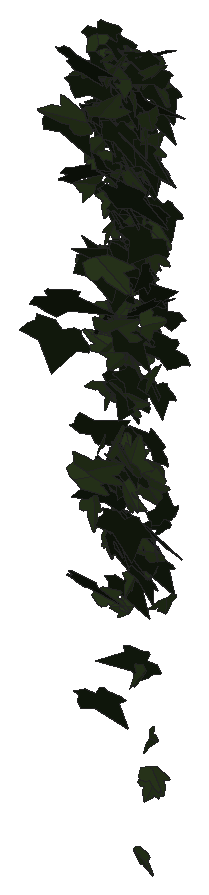
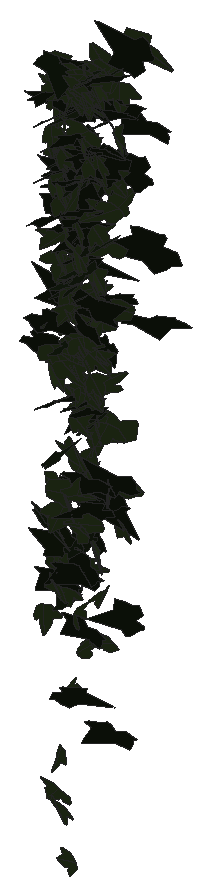
# SketchUp Ruby script. Lengths in millimetres.
U = 1.mm
M = Sketchup.active_model
def pt(a) = Geom::Point3d.new(a.map { |v| v * U })
def face(e, loops, mat)
  f = e.add_face(loops[0].map { |a| pt(a) })
  loops[1..].each { |l| e.add_face(l.map { |a| pt(a) }).erase! }
  f.material = f.back_material = mat if mat
  f
end
# faces: each face lists its corners as indices into pts; further lists are holes
def faces(e, pts, list, mat = nil) = list.each { |f| face(e, (f[0].is_a?(Array) ? f : [f]).map { |l| l.map { |i| pts[i] } }, mat) }
# xy, xz, yz: faces in a plane at the given z, y or x. An outline is a flat list of corners, or four numbers for a rectangle; further outlines are holes
def ring(l) = l.size == 4 ? [[l[0], l[1]], [l[2], l[1]], [l[2], l[3]], [l[0], l[3]]] : l.each_slice(2).to_a
def flat(e, list, mat, &to3) = list.each { |f| face(e, (f[0].is_a?(Array) ? f : [f]).map { |l| ring(l).map { |u, v| to3.(u, v) } }, mat) }
def xy(e, z, list, mat = nil) = flat(e, list, mat) { |x, y| [x, y, z] }
def xz(e, y, list, mat = nil) = flat(e, list, mat) { |x, z| [x, y, z] }
def yz(e, x, list, mat = nil) = flat(e, list, mat) { |y, z| [x, y, z] }
def lines(e, pts, list) = list.each { |a, b| e.add_line(pt(pts[a]), pt(pts[b])) }
# prism: a flat outline (further loops are holes) pulled along v
def prism(e, loops, v, mat = nil)
  f = face(e, loops, mat); d = Geom::Vector3d.new(v.map { |x| x * U })
  f.pushpull(f.normal.samedirection?(d) ? d.length : -d.length)
end
def box(e, o, s, mat = nil) = prism(e, [[o, [o[0] + s[0], o[1], o[2]], [o[0] + s[0], o[1] + s[1], o[2]], [o[0], o[1] + s[1], o[2]]]], [0, 0, s[2]], mat)
def at(x, y, z, deg = 0) = Geom::Transformation.translation(pt([x, y, z])) * Geom::Transformation.rotation(ORIGIN, Z_AXIS, deg.degrees)
def axes(o, x, y, z) = Geom::Transformation.new([*x, 0, *y, 0, *z, 0, *pt(o).to_a, 1])
def part(name) = M.definitions.add(name)
# library, detail: a bought-in or finely detailed component or shape, given as its bounding box
def library(name, o, s) = part(name).tap { |d| box(d.entities, o, s) }
def detail(e, o, s) = box(e.add_group.entities, o, s)
def put(e, d, t, mat = nil) = e.add_instance(d, t).tap { |i| i.material = mat if mat }
def group(e, t, mat = nil) = e.add_group.tap { |g| g.transformation = t; g.material = mat if mat }.entities
root = M.entities
M.materials.add("efeu1").color = [18, 25, 13]
M.materials.add("efeu2").color = [43, 57, 29]
c1 = part("ivyleaf_9")
p = [[39.1,54.8,31.7],[34.5,51.8,30.2],[-5.3,25.2,17.3],[-17.9,28.3,20.9],[-21.6,21.7,17],[-20.2,4.3,5.3],
  [-22.9,-0.3,2.5],[-17.1,-4,-0.6],[-2,-2.1,-1.2],[-0.7,-15.4,-10.1],[16.6,-22.3,-16.7],[21.1,-15.1,-12.5],
  [32.7,-10.7,-11],[46.1,-1.8,-6.6],[30.8,11.2,3.8]]
faces(c1.entities,p,[[0,1,2,3,4,5,6,7,8,9,10,11,12,13,14]],"efeu1")
c2 = part("ivyleaf_10")
p = [[0,12.8,-0.8],[-1.5,51.3,-10.9],[-4.9,51,-11.6],[-13.6,26.5,-7.3],[-13.2,15.9,-4.6],[-21.1,19.3,-7.2],
  [-29.5,16.3,-8.3],[-29.2,8.3,-6.2],[-19.7,-9.8,0.5],[-7.6,-13,4],[1,-12.2,5.8],[-0.4,51.1,-11.1],
  [-1.5,51.1,-10.9],[1,-12.4,5.9],[16.9,-12.4,3.5],[35.1,9.1,-5.1],[35,12.9,-6.1],[20.5,16.4,-4.9],
  [15.8,15,-3.8],[15.3,27.6,-7.1],[12.8,31.3,-7.8]]
faces(c2.entities,p,[[0,1,2,3,4,5,6,7,8,9,10],[11,12,0,13,14,15,16,17,18,19,20]],"efeu2")
put(root,c1,axes([1553.2,964.1,820.5],[-0.50844,0.05858,0.77802],[1.40559,-0.24621,0.27213],[0.47885,0.7849,0.02729]))
put(root,c2,axes([1579.3,950.2,1427.7],[-0.24843,-0.69259,0.43871],[-0.02175,-0.44266,-0.70222],[1.56018,-0.11645,0.06007]))
put(root,c2,axes([1577,960.7,824.2],[0.33546,-0.65964,-0.42013],[0.02498,0.43311,-0.6745],[1.48823,0.14142,0.10602]))
put(root,c1,axes([1546.8,926.5,544.2],[1.31033,-0.2504,0.31362],[0.56981,-0.09424,-0.7325],[0.50862,0.75066,0.01266]))
put(root,c2,axes([1580.3,922.5,1594.3],[-0.565,-0.7823,-0.20791],[0.09233,0.20386,-0.83633],[1.5378,-0.29967,-0.02617]))
put(root,c2,axes([1573.2,980.5,613.6],[0.08437,0.74047,-0.08975],[-0.02204,-0.08921,-0.74177],[-1.4194,0.0454,0.00618]))
put(root,c2,axes([1580,985.8,1246.2],[0.21882,-0.71346,0.22089],[0.15293,-0.21038,-0.72134],[1.4132,0.13324,0.04385]))
put(root,c1,axes([1569.5,984.6,1311.2],[-0.05011,-0.74368,0.2109],[-0.00636,-0.21091,-0.74413],[1.47117,-0.02624,0.00397]))
put(root,c2,axes([1587.5,986.1,1080.6],[-0.54365,-0.54241,0.47693],[-0.09608,-0.49662,-0.59505],[1.37126,-0.24984,0.14739]))
put(root,c2,axes([1576.9,950,1631.2],[0.52706,0.80701,-0.11706],[-0.07471,-0.11029,-0.8532],[-1.55018,0.2797,0.00132]))
put(root,c2,axes([1553.1,947.1,1170.7],[0.32062,-0.03138,-0.82619],[1.5099,0.24348,0.15252],[0.44293,-0.80727,0.07812]))
put(root,c2,axes([1578.4,932.1,1503.4],[0.49586,-0.68935,0.42023],[0.32415,-0.3847,-0.73667],[1.50195,0.31061,0.02025]))
put(root,c2,axes([1587.8,921.2,1357],[-0.25254,-0.35305,-0.84263],[-0.52564,-0.79613,0.37706],[-1.65742,0.30628,0.00881]))
put(root,c2,axes([1563,971.4,1378.3],[0.66493,0.37712,0.69187],[0.69454,0.59333,-0.50769],[-1.32915,0.4987,0.08083]))
put(root,c2,axes([1594.5,961.7,1014.7],[0.50491,0.5468,0.55529],[-0.49909,-0.48974,0.60754],[1.3967,-0.37267,0.01636]))
put(root,c1,axes([1607.6,969.1,1162.5],[0.25194,0.01031,0.85113],[-1.24923,0.54964,0.09543],[-1.03139,-0.6632,0.09232]))
put(root,c1,axes([1581.6,836.9,1095.2],[-1.20945,-0.79383,-0.19057],[0.21871,0.15212,-1.01684],[1.53827,-0.64577,-0.00526]))
put(root,c2,axes([1581.3,963.3,931],[-1.14052,-0.32781,-0.19698],[0.35024,0.07381,-0.68269],[0.63805,-0.62647,0.02264]))
put(root,c1,axes([1553.1,970.7,1466.3],[0.51611,-0.04869,0.76965],[1.46731,-0.00217,-0.27178],[0.0347,0.81602,0.0452]))
put(root,c1,axes([1565.5,966.3,1642.5],[0.4766,-0.57612,-0.54841],[0.17839,0.59232,-0.57945],[1.50328,0.11237,0.24263]))
put(root,c2,axes([1589.3,978.5,1474.5],[0.98995,-0.60809,-0.19504],[-0.1747,0.17774,-0.79897],[1.20277,0.52631,0.04448]))
put(root,c2,axes([1589.2,991.4,1471.5],[-0.44788,-0.6787,0.35841],[0.07888,-0.38557,-0.70291],[1.45861,-0.18755,0.14807]))
put(root,c2,axes([1590,984.7,1035],[-0.28456,-0.65758,0.24603],[0.0679,-0.25834,-0.6688],[1.33451,-0.12707,0.08649]))
put(root,c1,axes([1568.6,867.1,1511],[-0.737,-0.30191,-0.75298],[1.19702,0.41527,-0.48996],[0.97519,-0.7379,0.03234]))
put(root,c1,axes([1568.7,953.4,1464],[0.3838,-0.72001,0.34686],[0.20512,-0.32996,-0.7476],[1.50715,0.22826,0.01342]))
put(root,c1,axes([1583.5,960.1,1566.2],[-0.94398,-0.62896,-0.24306],[0.52877,0.08431,-0.7851],[1.16932,-0.54588,0.1588]))
put(root,c1,axes([1583.7,955.7,1478.7],[-0.03506,-0.05644,-0.837],[-0.2835,0.82412,-0.05229],[1.57123,0.14744,-0.02811]))
put(root,c1,axes([1598.6,934,1079.1],[-0.24507,0.18977,-0.77358],[-0.84612,0.63308,0.22931],[1.25782,0.46284,0.00353]))
put(root,c1,axes([1572.3,925.3,1566],[0.02901,-0.50716,-0.691],[0.44121,0.66779,-0.48501],[1.57051,-0.17824,0.14902]))
put(root,c1,axes([1600.9,977.5,1487.8],[-1.31585,-0.39869,-0.02994],[0.05183,0.01271,-0.7981],[0.75915,-0.69192,0.00259]))
put(root,c2,axes([1590.2,987.3,1232],[0.69057,-0.62123,0.21782],[0.24818,-0.17596,-0.71907],[1.22807,0.38489,0.02283]))
put(root,c1,axes([1596.7,965,1573.2],[-1.15022,0.19155,-0.52821],[0.90732,-0.23575,-0.63095],[-0.56593,-0.76726,0.062]))
put(root,c1,axes([1586,942.6,1186.7],[-0.56208,-0.69787,-0.3868],[0.30295,0.35262,-0.75775],[1.48803,-0.3354,0.00816]))
put(root,c2,axes([1600.1,965.1,1021.2],[-0.11367,-0.75429,-0.11919],[-0.00411,0.11972,-0.75657],[1.45337,-0.05865,-0.01146]))
put(root,c2,axes([1576.4,964.1,504.5],[0.62169,0.15414,0.55252],[0.96784,0.21635,-0.361],[-0.50507,0.60429,-0.01168]))
put(root,c2,axes([1598.7,965.3,1321.1],[-0.33191,-0.69901,0.42648],[0.25172,-0.45437,-0.69063],[1.53796,-0.07649,0.20507]))
put(root,c1,axes([1623,919.6,748.2],[0.27685,0.2147,-0.77453],[-1.16137,-0.48277,-0.24843],[-0.99555,0.62289,0.07443]))
put(root,c2,axes([1605.4,962.5,682.3],[0.51237,-0.70867,-0.2343],[-0.13007,0.22463,-0.75793],[1.41458,0.27734,0.01517]))
put(root,c1,axes([1582.4,938.5,313.9],[-0.39926,-0.28706,-0.70219],[0.86109,0.53744,-0.35488],[1.15888,-0.49824,0.02177]))
put(root,c1,axes([1580.3,863.4,1400.3],[0.82813,0.28551,0.7271],[1.10861,0.43596,-0.51978],[-0.99056,0.72661,0.02615]))
put(root,c2,axes([1600.3,956.8,930.8],[0.21076,-0.64099,0.29187],[0.2427,-0.27233,-0.64645],[1.3183,0.15261,0.07235]))
put(root,c2,axes([1609.4,949,934],[0.27722,-0.65135,-0.4833],[-0.15926,0.47634,-0.6672],[1.53539,0.16701,0.01806]))
put(root,c2,axes([1589.3,914,718.5],[1.1356,-0.55738,0.47425],[0.7327,-0.28134,-0.81501],[1.18453,0.70837,0.04947]))
put(root,c2,axes([1605.6,947,1606.8],[0.10812,-0.77024,0.32291],[0.09844,-0.31979,-0.7719],[1.58649,0.07234,0.02589]))
put(root,c2,axes([1616.9,969.9,996.7],[-0.73479,-0.51485,0.3183],[-0.34051,-0.2636,-0.64339],[1.10053,-0.42531,0.01345]))
put(root,c1,axes([1592.6,973.9,1472.6],[0.16464,-0.80557,0.01218],[0.00235,-0.01211,-0.8102],[1.53334,0.08652,-0.00006]))
put(root,c2,axes([1630.4,979.7,1096.7],[0.75171,-0.17944,-0.69683],[-1.24607,0.24014,-0.43294],[0.56811,0.76413,-0.02757]))
put(root,c2,axes([1612.2,970,1591.3],[-0.02635,-0.80711,0.4035],[-0.00876,-0.40348,-0.80722],[1.71733,-0.01444,0.00207]))
put(root,c2,axes([1616.8,986,1100],[-0.76549,-0.60764,0.20664],[-0.07645,-0.21955,-0.7238],[1.2191,-0.39531,0.08436]))
put(root,c1,axes([1600.4,984,1481.4],[-0.26422,-0.73324,-0.31717],[0.11325,0.31154,-0.74627],[1.51625,-0.15104,0.00047]))
put(root,c1,axes([1600.9,940.2,1389.8],[0.97713,-0.572,-0.38851],[0.46233,-0.30384,0.76836],[-1.23211,-0.56764,-0.01979]))
put(root,c2,axes([1612.9,977.1,1491.4],[0.2337,-0.78308,0.1817],[0.08478,-0.17689,-0.79248],[1.52759,0.12962,0.01619]))
put(root,c1,axes([1600,985.4,831.8],[-0.84978,-0.38149,-0.55998],[0.84482,0.34199,-0.58692],[0.9743,-0.62927,0.02051]))
put(root,c2,axes([1614.3,983.7,483.8],[-0.11398,0.22654,0.64254],[0.05682,-0.64352,0.22967],[1.29541,0.04816,0.04646]))
put(root,c1,axes([1615.8,993.5,1366.7],[-0.89601,-0.62643,0.13661],[-0.07365,-0.14141,-0.7818],[1.21801,-0.46937,0.05322]))
put(root,c1,axes([1597.5,985.1,1119.6],[-0.23735,0.33391,0.7135],[0.4991,-0.66359,0.35639],[1.41377,0.29033,-0.00603]))
put(root,c2,axes([1585.3,892.4,774.8],[1.09651,-0.02285,-0.69861],[1.33007,0.03606,0.57517],[0.02531,-0.90482,0.04057]))
put(root,c1,axes([1594,963,764.3],[0.59115,-0.12908,-0.7501],[0.13594,0.81153,-0.11007],[1.44219,-0.02358,0.31784]))
put(root,c1,axes([1610.4,962,1161.5],[-0.6732,-0.80074,-0.03054],[0.01734,0.02937,-0.87538],[1.52498,-0.35382,-0.00353]))
put(root,c1,axes([1631.8,974.6,1325.7],[-1.30354,-0.48834,0.22532],[0.35418,0.1271,0.84118],[-0.96034,0.70974,0.00439]))
put(root,c2,axes([1613.8,986.3,1085.1],[0.63108,-0.62278,0.27121],[0.21983,-0.24571,-0.70544],[1.27396,0.3509,-0.01262]))
put(root,c2,axes([1601.1,987,1016.6],[0.09106,-0.16675,0.7924],[0.98663,-0.60348,-0.1583],[1.1839,0.51575,0.07098]))
put(root,c1,axes([1580.5,868.7,1631.3],[1.50176,-0.0583,-0.62726],[1.19893,0.06764,0.78617],[-0.00643,-1.00574,0.08923]))
put(root,c2,axes([1629.4,959.1,1585.1],[-1.33031,0.40267,0.24094],[-0.5211,0.00109,-0.79612],[-0.72529,-0.73935,0.13005]))
put(root,c2,axes([1636.3,965.2,1186.4],[0.90924,0.37209,0.62338],[-0.92786,-0.38852,0.60553],[1.0238,-0.68256,-0.00485]))
put(root,c2,axes([1624.6,988.8,948],[-0.22543,-0.66028,0.3021],[-0.08533,-0.29885,-0.67078],[1.3793,-0.1264,0.00788]))
put(root,c1,axes([1619.6,985.2,1423.6],[-0.71336,-0.54248,0.44884],[-0.14077,-0.47533,-0.63626],[1.33261,-0.3406,0.17306]))
put(root,c1,axes([1608.1,969.4,959.2],[0.19809,-0.56039,-0.59148],[-0.17078,0.58477,-0.56983],[1.54128,0.13682,0.01288]))
put(root,c2,axes([1633.3,960.2,633.2],[0.21974,0.10985,-0.6521],[-0.87337,-0.46333,-0.1593],[-0.90622,0.47317,-0.0046]))
put(root,c1,axes([1592.5,930.3,788],[0.03445,-0.01786,-0.80652],[1.47555,0.22335,0.01245],[0.42434,-0.77519,0.02217]))
put(root,c2,axes([1623.1,948.1,1381.1],[0.07206,-0.88419,0.20304],[0.08956,-0.20103,-0.88421],[1.72426,0.04739,0.03744]))
put(root,c1,axes([1604.2,992.1,1243.3],[0.28876,-0.70872,0.27536],[0.13097,-0.26683,-0.7247],[1.44112,0.16626,0.01069]))
put(root,c2,axes([1600.3,968.6,734.4],[0.14711,0.08817,0.65436],[0.90398,0.45022,-0.11677],[-0.87291,0.48111,-0.01065]))
put(root,c1,axes([1603,968.1,938.2],[0.5348,-0.79613,0.03812],[0.02513,-0.03576,-0.84426],[1.51672,0.28131,0.00055]))
put(root,c1,axes([1605.4,930.8,1611.6],[0.36961,-0.86612,-0.10074],[-0.00509,0.10262,-0.88741],[1.65951,0.19322,0.01972]))
put(root,c1,axes([1599.8,986.6,661.2],[-0.16013,-0.06326,-0.801],[1.52841,-0.03262,-0.08178],[-0.04936,-0.80475,0.06628]))
put(root,c2,axes([1633.9,956.6,1070.4],[0.15444,0.10556,-0.80531],[-0.80032,-0.68695,-0.13241],[-1.32248,0.42804,-0.01391]))
put(root,c1,axes([1599.3,966.9,1449.7],[-0.32944,-0.19482,-0.78981],[1.35547,0.35389,-0.24339],[0.74812,-0.72699,0.09318]))
put(root,c1,axes([1609.3,968.9,1197.3],[0.11046,-0.8437,0.16627],[0.02176,-0.16588,-0.84569],[1.63647,0.05916,0.00002]))
put(root,c2,axes([1627.8,976.7,795.4],[0.75353,0.71423,-0.06043],[0.04288,0.0566,0.81659],[1.36351,-0.39649,0.00771]))
put(root,c2,axes([1631.3,981.2,1330.1],[0.71497,-0.66326,-0.23099],[-0.09882,0.23501,-0.75926],[1.33303,0.37317,0.06761]))
put(root,c1,axes([1659.9,926.3,1223.8],[-0.58858,-0.24955,-0.7248],[-1.0734,-0.45524,0.39738],[-0.98805,0.64322,0.00005]))
put(root,c1,axes([1609.3,967.4,1629.8],[0.78641,-0.65407,-0.35834],[-0.04534,0.39788,-0.75371],[1.41868,0.37529,0.17455]))
put(root,c1,axes([1609.2,982.7,532.4],[-0.52358,-0.15245,-0.73315],[1.31351,0.25147,-0.31126],[0.55304,-0.74159,0.04517]))
put(root,c1,axes([1651.6,985.9,385.7],[-0.21632,-0.23589,-0.72644],[-0.57885,-0.65972,0.26181],[-1.3334,0.32466,0.0042]))
put(root,c2,axes([1628.5,978,1271.5],[0.15272,-0.74492,0.4313],[0.28988,-0.41405,-0.74346],[1.61237,0.145,0.09281]))
put(root,c1,axes([1617.6,967.3,1309.9],[0.25135,-0.23624,-0.7395],[-0.08144,0.74676,-0.2462],[1.47523,0.08148,0.11241]))
put(root,c2,axes([1642.4,925.1,1080.2],[-0.8731,0.62383,-0.26821],[-0.29832,0.21765,0.77435],[1.25745,0.48479,-0.00252]))
put(root,c1,axes([1606.4,980.4,1382],[0.38777,-0.39841,0.65952],[0.61247,-0.57584,-0.44727],[1.33242,0.38064,0.01366]))
put(root,c2,axes([1644.2,963.5,1615.1],[-1.20418,-0.46629,0.31865],[-0.31944,-0.30164,-0.77468],[1.02631,-0.64099,0.13275]))
put(root,c2,axes([1635.2,946,1621.7],[0.32124,-0.82107,0.0643],[0.0173,-0.06378,-0.83823],[1.56735,0.16899,-0.00393]))
put(root,c2,axes([1653.7,982.8,1038.5],[-0.9763,-0.12537,0.52481],[-0.92748,-0.20321,-0.52489],[0.44085,-0.70518,0.05795]))
put(root,c2,axes([1628.5,981.2,548.2],[-0.04967,-0.41174,0.64745],[0.48097,-0.61629,-0.38174],[1.3788,0.20015,0.15649]))
put(root,c2,axes([1640.1,914.6,1613.1],[-0.0196,-0.84798,0.00435],[-0.00129,-0.00435,-0.84804],[1.61389,-0.0103,-0.00063]))
put(root,c2,axes([1640.8,972.1,1252.8],[0.88057,-0.51593,-0.37367],[-0.1984,0.39428,-0.67347],[1.19607,0.44525,0.16339]))
put(root,c2,axes([1634.2,968.2,1386.3],[-0.10188,-0.46642,-0.73818],[0.39148,0.71201,-0.4648],[1.61507,-0.20201,0.0661]))
put(root,c2,axes([1641.8,944.4,1077.2],[-1.58503,-0.24757,-0.02247],[0.04099,0.0064,-0.86884],[0.47133,-0.8331,0]))
put(root,c1,axes([1623.5,978.5,1487.1],[-0.65072,-0.01316,-0.75416],[1.42996,-0.07885,-0.33926],[-0.12641,-0.82428,0.04449]))
put(root,c2,axes([1678,767,1587.8],[-0.60878,0.03576,1.02162],[-1.94483,-0.04001,-0.31855],[0.05238,-1.06978,0.04607]))
put(root,c2,axes([1617.9,972.5,1517.2],[1.26709,-0.04122,0.48485],[0.92497,0.09693,-0.65911],[-0.04576,0.81788,0.10255]))
put(root,c2,axes([1624.6,979.8,998.5],[-0.3606,0.35478,-0.70623],[0.63363,-0.62283,-0.40221],[-1.3642,-0.38307,-0.00013]))
put(root,c2,axes([1654,979.5,1607.1],[1.20615,-0.1704,-0.49947],[-0.78431,0.32779,-0.63472],[0.62742,0.73733,0.16674]))
put(root,c1,axes([1611.5,772.8,1201.2],[0.24918,0.34043,-0.9819],[0.79136,0.88983,0.36395],[1.81266,-0.43528,-0.02391]))
put(root,c2,axes([1660.5,910.2,1602.6],[0.85904,-0.30497,-0.6524],[-0.9588,0.41648,-0.54324],[0.97942,0.6752,0.04041]))
put(root,c2,axes([1641.9,980.5,1592.2],[1.40456,-0.35805,-0.05001],[-0.08358,0.02405,-0.82027],[0.68296,0.7393,0.00247]))
put(root,c2,axes([1622.3,976.2,715.1],[-0.13213,-0.02924,-0.7553],[0.92616,-0.58211,-0.02219],[-1.10077,-0.48626,0.07199]))
put(root,c1,axes([1623.8,979.9,635.6],[-0.31742,-0.29222,-0.73956],[0.8585,0.58754,-0.33388],[1.24636,-0.47912,0.04163]))
put(root,c1,axes([1643.8,958.9,783.2],[-0.7189,-0.71163,0.2055],[-0.13587,-0.19463,-0.8052],[1.40315,-0.38345,0.02732]))
put(root,c1,axes([1631.2,970.5,1226.8],[0.11376,-0.8047,-0.22714],[-0.03266,0.22649,-0.80692],[1.59101,0.06219,-0.00032]))
put(root,c1,axes([1622.7,963.1,1280.4],[0.76678,-0.6896,0.17223],[0.15489,-0.15191,-0.79864],[1.34387,0.41098,-0.00622]))
put(root,c1,axes([1626.6,974.1,1505.4],[0.08748,-0.61099,-0.5297],[0.36788,0.52347,-0.58704],[1.49438,-0.0931,0.17552]))
put(root,c1,axes([1632.3,956.4,1618.5],[1.42832,-0.24329,-0.31092],[-0.48255,0.21488,-0.78015],[0.57594,0.78341,0.11743]))
put(root,c2,axes([1649.6,897.4,850.3],[0.40428,-0.57349,0.74298],[-0.51097,0.69281,0.61152],[-1.71163,-0.34228,-0.00707]))
put(root,c2,axes([1672.7,975,1042.1],[-0.76065,-0.02559,0.65672],[-1.20741,-0.18571,-0.39333],[0.32666,-0.74601,0.07539]))
put(root,c2,axes([1651.6,985.9,1468],[-0.32374,-0.70333,0.36719],[0.06803,-0.38194,-0.71503],[1.50848,-0.13372,0.11105]))
put(root,c2,axes([1678,979.3,780.7],[-0.07269,0.01051,-0.82546],[-1.54899,-0.13874,0.03589],[-0.26287,0.81461,0.01677]))
put(root,c1,axes([1640.9,963.2,1310.9],[0.91706,-0.45178,-0.49466],[-0.66356,0.35118,-0.66037],[1.0887,0.59459,0.01418]))
put(root,c2,axes([1655.2,972.3,1176.7],[-0.43933,-0.72927,-0.11946],[0.03344,0.1197,-0.76469],[1.40605,-0.23071,-0.01914]))
put(root,c1,axes([1643.1,992.9,1209.5],[-0.45582,-0.64663,0.41145],[0.13306,-0.44771,-0.66292],[1.4526,-0.1619,0.18983]))
put(root,c2,axes([1659.8,963.3,1588.5],[1.5221,0.09118,0.33671],[-0.63548,-0.04369,0.80492],[0.19218,-0.86665,-0.00516]))
put(root,c2,axes([1656,977.7,772.2],[0.4812,-0.70242,-0.14184],[-0.09026,0.13368,-0.74654],[1.36084,0.25725,0.00064]))
put(root,c1,axes([1635.1,975.8,1234.9],[0.56442,-0.74638,-0.0655],[-0.02321,0.06563,-0.80304],[1.42579,0.29654,0.01286]))
put(root,c2,axes([1665.6,924.7,808.1],[-1.48469,0.3793,-0.22604],[-0.38705,0.09867,0.86743],[0.74591,0.80617,0.00019]))
put(root,c2,axes([1643.6,977.1,1156.6],[0.41932,0.6973,0.28447],[0.17261,0.26967,-0.73126],[-1.42286,0.23821,-0.00488]))
put(root,c1,axes([1640.3,950.1,817.7],[0.03985,-0.78271,0.14834],[0.04427,-0.14772,-0.78276],[1.51553,0.02489,0.01897]))
put(root,c1,axes([1653.2,951.3,947.5],[-0.65334,-0.71894,0.30983],[-0.18093,-0.29752,-0.79571],[1.47891,-0.35401,0.03953]))
put(root,c2,axes([1672,963.6,1045.5],[0.33579,-0.33255,-0.74052],[-0.74684,0.62845,-0.37572],[1.35245,0.4296,-0.02362]))
put(root,c1,axes([1644.9,947.8,1238],[-0.26825,-0.68707,-0.3531],[0.17954,0.34093,-0.70106],[1.45921,-0.16826,0.02135]))
put(root,c2,axes([1654.2,959,1578.3],[-0.503,0.78796,0.1323],[-0.07117,0.127,-0.83109],[-1.51898,-0.26688,-0.00487]))
put(root,c2,axes([1662.9,963.5,1362.3],[0.84143,-0.51866,-0.50472],[-0.24893,0.52445,-0.6535],[1.35468,0.41852,0.19342]))
put(root,c1,axes([1641.4,949.8,1546.1],[1.07185,-0.38083,-0.47393],[-0.32502,0.52092,-0.62152],[1.11051,0.52003,0.27552]))
put(root,c1,axes([1642.1,969.4,1201.3],[0.76448,-0.62268,-0.23895],[-0.18229,0.2222,-0.74002],[1.25619,0.41119,0.03803]))
put(root,c1,axes([1644.2,918.8,1493.4],[0.15735,-0.80664,-0.15809],[0.00555,0.15917,-0.81065],[1.56439,0.08057,0.01878]))
put(root,c1,axes([1637.4,965,681.2],[0.96019,-0.6398,0.07736],[0.08146,-0.06476,-0.81476],[1.22383,0.50629,-0.00646]))
put(root,c2,axes([1652.7,969.8,1289.4],[0.68909,-0.74021,0.06166],[0.04119,0.07908,0.82225],[-1.41306,-0.35867,0.05404]))
put(root,c2,axes([1666.5,977.9,1362.5],[-0.50005,-0.66612,0.34597],[0.00316,-0.36707,-0.70548],[1.42854,-0.23236,0.12266]))
put(root,c2,axes([1658.9,982.9,590],[1.26747,0.04095,-0.03859],[-0.07329,-0.00251,-0.66722],[-0.07809,0.66708,-0.00014]))
put(root,c2,axes([1647.4,900.5,1089.9],[-1.22102,-0.45455,0.48942],[0.75694,0.28524,0.78626],[-1.02131,0.75483,-0.00239]))
put(root,c1,axes([1653.2,976.2,1321.1],[-0.2934,-0.76532,-0.13074],[0.07019,0.12592,-0.78061],[1.47599,-0.15812,0.01113]))
put(root,c1,axes([1661.9,965.7,966.2],[-0.69913,-0.70354,0.23615],[-0.11199,-0.23505,-0.79181],[1.40794,-0.36805,0.05428]))
put(root,c1,axes([1648.6,972.8,1389.6],[-0.08007,-0.69428,0.40959],[0.22349,-0.41105,-0.6847],[1.5178,0.0239,0.12243]))
put(root,c2,axes([1690.9,962.5,630.8],[-0.42785,-0.07761,0.73543],[-1.34169,-0.20971,-0.23762],[0.42517,-0.73988,-0.00979]))
put(root,c1,axes([1651.8,990.3,1079.5],[-0.03671,-0.6741,0.36436],[0.10282,-0.36476,-0.67199],[1.45473,0.00877,0.05669]))
put(root,c2,axes([1672.5,969.1,1621.4],[-1.02,-0.62148,0.1296],[-0.0954,-0.12765,-0.81943],[1.20448,-0.53641,0.04485]))
put(root,c2,axes([1641.1,934.1,934.5],[-0.97697,-0.02017,0.73254],[1.39224,-0.06717,0.51077],[0.08275,0.89197,0.05503]))
put(root,c1,axes([1643.6,904.2,670.2],[-0.04016,-0.1428,-0.81049],[1.5206,-0.19793,0.01407],[-0.37552,-0.78623,0.14366]))
put(root,c2,axes([1661.5,962.8,373.4],[0.03585,-0.12677,0.74134],[0.44199,-0.70435,-0.12635],[1.36145,0.232,0.0215]))
put(root,c1,axes([1651.6,977.8,566.5],[0.14524,-0.69201,0.33747],[0.14034,-0.33099,-0.69541],[1.45856,0.10075,0.03331]))
put(root,c2,axes([1670.8,974.6,1394.6],[0.03972,-0.80675,0.00868],[-0.00152,-0.00871,-0.80702],[1.5355,0.02086,-0.00102]))
put(root,c1,axes([1652.8,934,1555.1],[0.11208,-0.76881,0.33445],[0.10598,-0.33094,-0.77057],[1.59214,0.07615,0.02775]))
put(root,c2,axes([1666.1,979,745],[-1.05928,-0.53977,-0.29898],[0.41649,0.20379,-0.77531],[1.09802,-0.59803,0.00565]))
put(root,c1,axes([1643.8,941,1470.6],[0.71265,-0.72279,0.32065],[0.30653,-0.27762,-0.8139],[1.47335,0.40737,0.01424]))
put(root,c2,axes([1640.5,945.5,1398.1],[0.07878,-0.15368,0.89806],[1.54866,-0.39818,-0.10565],[0.78007,0.80602,0.11904]))
put(root,c2,axes([1672,981.4,1453.9],[0.81628,-0.68381,-0.07997],[-0.06248,0.0738,-0.8071],[1.3088,0.43,0.01134]))
put(root,c2,axes([1674.7,951.6,1450.4],[-1.49105,-0.3182,-0.0267],[0.04684,0.01037,-0.8456],[0.60593,-0.78383,-0.00035]))
put(root,c1,axes([1675.4,968,1629.4],[0.52012,0.79502,0.12704],[-0.00431,0.13492,-0.83945],[-1.53227,0.26949,0.04549]))
put(root,c2,axes([1686.7,976.1,1056.2],[-1.21907,-0.16917,0.35413],[-0.64062,-0.11173,-0.66221],[0.38407,-0.72333,0.01947]))
put(root,c1,axes([1661.5,976.6,1402.9],[-0.3888,-0.7427,-0.23212],[0.14904,0.21915,-0.7701],[1.47341,-0.21815,0.01665]))
put(root,c2,axes([1674.4,922.1,1564.4],[0.83181,-0.59727,-0.40094],[-0.07193,0.44943,-0.7107],[1.3672,0.38703,0.20654]))
put(root,c1,axes([1691.5,945.7,1342.8],[0.58794,0.16969,-0.77235],[-1.31972,-0.34046,-0.35215],[-0.72345,0.75898,0.01472]))
put(root,c2,axes([1685.3,958.5,1043.2],[-1.22499,-0.20012,0.28154],[-0.47044,-0.14904,-0.67103],[0.4592,-0.68654,0.06361]))
put(root,c2,axes([1647.8,871.7,1237.6],[1.29185,0.4004,0.57075],[0.95125,0.27589,-0.78796],[-0.92507,0.84284,-0.01322]))
put(root,c2,axes([1648.6,964,1395.1],[-0.39558,0.02509,0.85234],[1.43525,-0.40407,0.1958],[0.75748,0.77872,0.07413]))
put(root,c2,axes([1676.9,960.2,1233.4],[-1.5714,0.06183,-0.04539],[0.08526,-0.00958,-0.82795],[-0.11849,-0.82685,0.0062]))
put(root,c2,axes([1680.6,952.4,1023.9],[0.21051,0.72226,0.03],[-0.10323,-0.02197,0.72895],[1.37191,-0.11248,0.05025]))
put(root,c2,axes([1675.2,963.9,1449],[0.38294,-0.74109,0.28245],[0.18295,-0.26646,-0.76761],[1.49828,0.22195,0.02154]))
put(root,c1,axes([1657.1,965.5,1429.5],[0.59718,-0.67534,-0.46793],[0.02883,0.50556,-0.7195],[1.56342,0.24864,0.192]))
put(root,c2,axes([1679.1,968.7,1246.9],[0.39726,-0.75785,0.03815],[0.01691,-0.03713,-0.78607],[1.44407,0.20892,-0.00129]))
put(root,c2,axes([1675.6,975.1,148.6],[1.06652,-0.4294,0.00961],[0.01517,-0.00539,-0.70598],[0.8173,0.56044,0.00057]))
put(root,c2,axes([1672.9,912.6,773.6],[-0.12678,0.81263,0.14964],[-0.02042,0.14926,-0.81535],[-1.57246,-0.06746,-0.00147]))
put(root,c1,axes([1662.3,901.4,658.3],[1.11034,-0.50657,-0.29355],[-0.38272,0.21582,-0.7721],[1.0465,0.61641,0.02909]))
put(root,c2,axes([1657.3,835.7,839.3],[-1.48722,-0.19509,0.63211],[1.1749,0.13657,0.8053],[-0.45251,0.99577,0.01339]))
put(root,c2,axes([1671,931.1,821.5],[1.49185,-0.56977,0.04211],[-0.06486,0.02474,0.96906],[-1.0854,-0.7846,-0.00002]))
put(root,c1,axes([1642.1,939.5,1542.4],[1.0584,-0.12227,0.71843],[1.33775,-0.14862,-0.56939],[0.36622,0.89627,0.00359]))
put(root,c2,axes([1674.1,844.9,1566.5],[-0.88722,-0.77023,0.19402],[0.1972,0.16408,0.90031],[-1.49878,0.47753,0.00361]))
put(root,c2,axes([1680.9,963.6,248.2],[0.02298,-0.43341,-0.60314],[0.16053,0.60012,-0.42955],[1.40438,-0.06151,0.05897]))
put(root,c2,axes([1677.5,988.6,1404.9],[0.0746,-0.65402,0.47141],[0.39134,-0.44825,-0.63899],[1.48364,0.15112,0.14484]))
put(root,c2,axes([1680.9,983.1,598],[0.656,-0.5933,0.12863],[0.10203,-0.1176,-0.68605],[1.1509,0.3486,-0.0125]))
put(root,c2,axes([1706.8,957.2,780.2],[0.09069,0.02788,0.68359],[-1.29566,0.06996,0.0446],[-0.12926,-0.68167,0.03253]))
put(root,c1,axes([1692.4,979.5,831.2],[0.13188,-0.84181,0.0159],[0.06813,0.01889,0.84384],[-1.60097,-0.06854,0.03722]))
put(root,c1,axes([1652.8,965.8,1413],[0.73222,-0.07551,-0.73353],[1.40012,-0.01756,0.38766],[-0.09645,-0.82812,0.05866]))
put(root,c1,axes([1670.9,910.9,1085.8],[0.2804,-0.72504,-0.4325],[-0.13414,0.42694,-0.73973],[1.60116,0.16274,0.01377]))
put(root,c1,axes([1704,951.9,1620.7],[-1.39488,-0.31909,0.29154],[-0.47331,-0.15809,-0.79821],[0.6728,-0.77277,0.04291]))
put(root,c1,axes([1705.8,977.6,1118.4],[0.08167,0.05635,-0.77252],[-0.67694,-0.68587,-0.06979],[-1.30955,0.35806,-0.0121]))
put(root,c2,axes([1674.7,942.4,22.1],[-0.49655,0.30336,-0.57071],[0.64357,-0.46044,-0.39933],[-1.04831,-0.42636,0.02517]))
put(root,c1,axes([1672,975,604.2],[-0.59958,-0.15948,-0.69624],[1.14583,0.35017,-0.35263],[0.73148,-0.67925,-0.01832]))
put(root,c2,axes([1676.3,981.3,629.7],[-0.02905,-0.09309,0.66356],[0.85189,-0.49533,-0.0592],[0.94897,0.44181,0.07345]))
put(root,c1,axes([1698.6,944.9,1277.3],[-1.1519,-0.52091,0.05023],[-0.08083,-0.02765,-0.79851],[0.9927,-0.6067,-0.00674]))
put(root,c1,axes([1683.9,981.3,957],[-0.15001,-0.76088,0.06984],[0.01374,-0.07095,-0.76481],[1.45412,-0.07782,0.01443]))
put(root,c1,axes([1663.1,902.4,1380.9],[-0.03161,-0.01432,-0.94426],[1.61316,0.41621,-0.02122],[0.79253,-0.84775,0.00553]))
put(root,c1,axes([1669.4,950.7,1155.9],[-0.16356,-0.06716,0.83269],[1.2792,-0.50267,0.02882],[0.9442,0.66939,0.10519]))
put(root,c2,axes([1679.6,972.4,175.2],[1.10001,-0.10428,0.39461],[0.73777,-0.0739,-0.5873],[0.24317,0.69593,-0.00323]))
put(root,c1,axes([1680.2,967.9,1527.8],[0.35913,-0.7555,-0.26525],[0.02795,0.27573,-0.77492],[1.52365,0.17302,0.07674]))
put(root,c2,axes([1683,947.9,1484.6],[0.46206,-0.5067,0.6357],[0.82064,-0.48216,-0.549],[1.31159,0.48018,0.11955]))
put(root,c1,axes([1690.1,948.7,1202.8],[0.01286,-0.30434,-0.73503],[0.93146,-0.57791,0.24379],[-1.19366,-0.45424,0.18232]))
put(root,c1,axes([1689.6,921.7,1141],[-0.13338,0.57851,-0.58892],[-0.14548,0.58396,0.58273],[1.56441,0.10363,0.00398]))
put(root,c2,axes([1684,960.4,1284.2],[0.668,0.57622,0.41951],[0.42983,0.35362,-0.67466],[-1.28662,0.4173,-0.00758]))
put(root,c1,axes([1684.5,949.8,1432],[0.16205,-0.79086,0.19974],[-0.0055,-0.20112,-0.79508],[1.55242,0.08184,-0.02367]))
put(root,c1,axes([1680.7,923.2,1462.9],[0.48484,-0.64378,-0.46681],[0.05742,0.49765,-0.66985],[1.51236,0.18749,0.17509]))
put(root,c2,axes([1676.4,968.2,1580.1],[1.24794,-0.09204,0.51456],[0.99386,0.07847,-0.65141],[0.04444,0.8298,0.11868]))
put(root,c2,axes([1700.6,957.4,1004.4],[0.20792,-0.81636,0.27169],[0.14935,-0.26328,-0.82263],[1.63066,0.1282,0.0407]))
put(root,c2,axes([1703.2,958.8,1481.8],[-0.32553,-0.76245,-0.18321],[0.09973,0.17598,-0.7813],[1.48906,-0.17847,0.01227]))
put(root,c1,axes([1712.9,963.7,708.6],[-1.01169,0.4474,-0.34863],[-0.5027,0.22758,0.69478],[0.9553,0.59357,-0.00361]))
put(root,c2,axes([1703.1,932,1535.4],[-0.60861,-0.81806,-0.31942],[0.21005,0.2998,-0.87832],[1.65815,-0.33824,-0.00598]))
put(root,c2,axes([1691.9,938.5,1103.5],[0.15339,-0.14337,-0.86405],[0.6839,0.79672,-0.09868],[1.52019,-0.34396,0.13158]))
put(root,c1,axes([1674.4,968.6,665.3],[0.57211,-0.52854,0.55192],[0.6446,-0.43951,-0.60536],[1.30374,0.44924,0.05711]))
put(root,c2,axes([1704.9,978.8,531.1],[-0.39168,-0.72629,-0.2237],[0.09514,0.21832,-0.75481],[1.44322,-0.2115,-0.01095]))
put(root,c2,axes([1708.5,951.3,1619.6],[-0.20272,-0.79215,0.30213],[-0.08916,-0.29854,-0.79925],[1.61108,-0.1162,-0.00622]))
put(root,c1,axes([1694,983.7,1323.9],[-0.1457,-0.78421,-0.09647],[-0.00826,0.09734,-0.78782],[1.50373,-0.07545,-0.01367]))
put(root,c1,axes([1724.3,961.6,705.9],[-0.85824,0.63568,0.03637],[-0.04014,0.02963,-0.77938],[-1.21113,-0.45144,0.00006]))
put(root,c1,axes([1735.2,961.5,1057.2],[-0.29745,-0.12747,-0.81514],[-1.18661,-0.52511,0.20166],[-1.02839,0.64277,0.00309]))
put(root,c1,axes([1694.1,974.6,1570],[-0.0937,-0.78415,-0.25934],[0.04301,0.25842,-0.78567],[1.5713,-0.05383,0.00604]))
put(root,c1,axes([1696.8,873.8,734.8],[-1.19715,-0.2297,-0.64286],[1.15392,0.21376,-0.66963],[0.5971,-0.87364,0.00518]))
